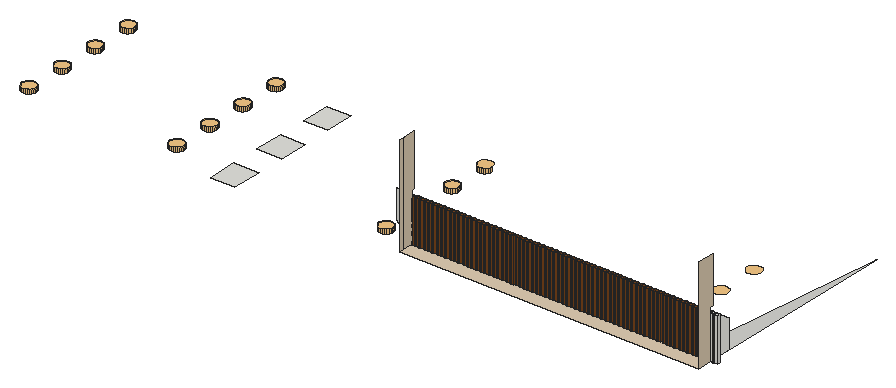
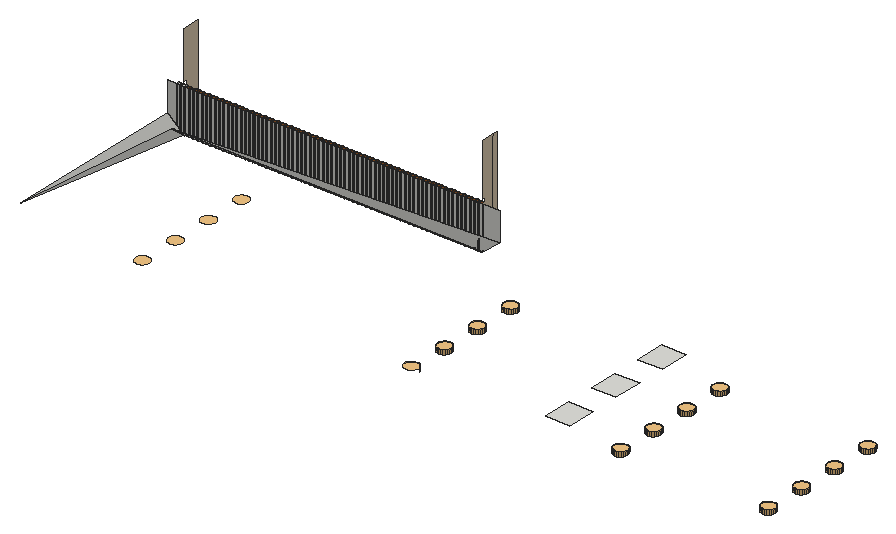
# SketchUp Ruby script. Lengths in inches.
U = 1.inch
M = Sketchup.active_model
def pt(a) = Geom::Point3d.new(a.map { |v| v * U })
def face(e, loops, mat)
  f = e.add_face(loops[0].map { |a| pt(a) })
  loops[1..].each { |l| e.add_face(l.map { |a| pt(a) }).erase! }
  f.material = f.back_material = mat if mat
  f
end
# faces: each face lists its corners as indices into pts; further lists are holes
def faces(e, pts, list, mat = nil) = list.each { |f| face(e, (f[0].is_a?(Array) ? f : [f]).map { |l| l.map { |i| pts[i] } }, mat) }
# xy, xz, yz: faces in a plane at the given z, y or x. An outline is a flat list of corners, or four numbers for a rectangle; further outlines are holes
def ring(l) = l.size == 4 ? [[l[0], l[1]], [l[2], l[1]], [l[2], l[3]], [l[0], l[3]]] : l.each_slice(2).to_a
def flat(e, list, mat, &to3) = list.each { |f| face(e, (f[0].is_a?(Array) ? f : [f]).map { |l| ring(l).map { |u, v| to3.(u, v) } }, mat) }
def xy(e, z, list, mat = nil) = flat(e, list, mat) { |x, y| [x, y, z] }
def xz(e, y, list, mat = nil) = flat(e, list, mat) { |x, z| [x, y, z] }
def yz(e, x, list, mat = nil) = flat(e, list, mat) { |y, z| [x, y, z] }
def lines(e, pts, list) = list.each { |a, b| e.add_line(pt(pts[a]), pt(pts[b])) }
# prism: a flat outline (further loops are holes) pulled along v
def prism(e, loops, v, mat = nil)
  f = face(e, loops, mat); d = Geom::Vector3d.new(v.map { |x| x * U })
  f.pushpull(f.normal.samedirection?(d) ? d.length : -d.length)
end
def box(e, o, s, mat = nil) = prism(e, [[o, [o[0] + s[0], o[1], o[2]], [o[0] + s[0], o[1] + s[1], o[2]], [o[0], o[1] + s[1], o[2]]]], [0, 0, s[2]], mat)
def at(x, y, z, deg = 0) = Geom::Transformation.translation(pt([x, y, z])) * Geom::Transformation.rotation(ORIGIN, Z_AXIS, deg.degrees)
def axes(o, x, y, z) = Geom::Transformation.new([*x, 0, *y, 0, *z, 0, *pt(o).to_a, 1])
def part(name) = M.definitions.add(name)
# library, detail: a bought-in or finely detailed component or shape, given as its bounding box
def library(name, o, s) = part(name).tap { |d| box(d.entities, o, s) }
def detail(e, o, s) = box(e.add_group.entities, o, s)
def put(e, d, t, mat = nil) = e.add_instance(d, t).tap { |i| i.material = mat if mat }
def group(e, t, mat = nil) = e.add_group.tap { |g| g.transformation = t; g.material = mat if mat }.entities
root = M.entities
M.materials.add("Generic\#1").color = [121, 68, 27]
M.materials.add("Generic\#2").color = [245, 199, 133]
M.materials.add("Generic\#6").color = [223, 205, 179]
c1 = part("Group\#11")
xy(c1.entities,26.3125,[[0,0,2,2]])
xz(c1.entities,0,[[0,0,2,26.3125]])
yz(c1.entities,0,[[0,0,2,26.3125]])
yz(c1.entities,2,[[0,0,2,26.3125]])
xy(root,122,[[190.6,57.81,205.29,75.37],[190.6,92.87,205.29,110.43],[190.6,127.93,205.29,145.49]])
xy(root,122.5625,[[68.07,68.72,66.98,68.86,65.97,69.28,65.11,69.95,64.44,70.8125,64.02,71.82,63.88,72.91,64.02,73.99,64.44,75,65.11,75.87,65.97,76.53,66.98,76.95,68.07,77.09,69.15,76.95,70.16,76.53,71.03,75.87,71.69,75,72.11,73.99,72.25,72.91,72.11,71.82,71.69,70.8125,71.03,69.95,70.16,69.28,69.15,68.86],[157.88,68.72,156.8,68.86,155.79,69.28,154.92,69.95,154.25,70.8125,153.83,71.82,153.69,72.91,153.83,73.99,154.25,75,154.92,75.87,155.79,76.53,156.8,76.95,157.88,77.09,158.96,76.95,159.97,76.53,160.84,75.87,161.51,75,161.92,73.99,162.07,72.91,161.92,71.82,161.51,70.8125,160.84,69.95,159.97,69.28,158.96,68.86],[284.88,68.72,283.8,68.86,282.79,69.28,281.92,69.95,281.25,70.8125,280.83,71.82,280.69,72.91,280.83,73.99,281.25,75,281.92,75.87,282.79,76.53,283.8,76.95,284.88,77.09,285.96,76.95,286.97,76.53,287.84,75.87,288.51,75,288.92,73.99,289.07,72.91,288.92,71.82,288.51,70.8125,287.84,69.95,286.97,69.28,285.96,68.86],[448.19,68.72,447.11,68.86,446.1,69.28,445.23,69.95,444.57,70.8125,444.15,71.82,444,72.91,444.15,73.99,444.57,75,445.23,75.87,446.1,76.53,447.11,76.95,448.19,77.09,449.28,76.95,450.29,76.53,451.15,75.87,451.82,75,452.24,73.99,452.38,72.91,452.24,71.82,451.82,70.8125,451.15,69.95,450.29,69.28,449.28,68.86],[68.07,93.78,66.98,93.92,65.97,94.34,65.11,95.01,64.44,95.875,64.02,96.89,63.88,97.97,64.02,99.05,64.44,100.0625,65.11,100.93,65.97,101.6,66.98,102.01,68.07,102.16,69.15,102.01,70.16,101.6,71.03,100.93,71.69,100.0625,72.11,99.05,72.25,97.97,72.11,96.89,71.69,95.875,71.03,95.01,70.16,94.34,69.15,93.92],
  [157.88,93.78,156.8,93.92,155.79,94.34,154.92,95.01,154.25,95.875,153.83,96.89,153.69,97.97,153.83,99.05,154.25,100.0625,154.92,100.93,155.79,101.6,156.8,102.01,157.88,102.16,158.96,102.01,159.97,101.6,160.84,100.93,161.51,100.0625,161.92,99.05,162.07,97.97,161.92,96.89,161.51,95.875,160.84,95.01,159.97,94.34,158.96,93.92],[284.88,93.78,283.8,93.92,282.79,94.34,281.92,95.01,281.25,95.875,280.83,96.89,280.69,97.97,280.83,99.05,281.25,100.0625,281.92,100.93,282.79,101.6,283.8,102.01,284.88,102.16,285.96,102.01,286.97,101.6,287.84,100.93,288.51,100.0625,288.92,99.05,289.07,97.97,288.92,96.89,288.51,95.875,287.84,95.01,286.97,94.34,285.96,93.92],[448.19,93.78,447.11,93.92,446.1,94.34,445.23,95.01,444.57,95.875,444.15,96.89,444,97.97,444.15,99.05,444.57,100.0625,445.23,100.93,446.1,101.6,447.11,102.01,448.19,102.16,449.28,102.01,450.29,101.6,451.15,100.93,451.82,100.0625,452.24,99.05,452.38,97.97,452.24,96.89,451.82,95.875,451.15,95.01,450.29,94.34,449.28,93.92],[68.07,118.84,66.98,118.99,65.97,119.41,65.11,120.07,64.44,120.9375,64.02,121.95,63.88,123.03,64.02,124.12,64.44,125.125,65.11,125.99,65.97,126.66,66.98,127.08,68.07,127.22,69.15,127.08,70.16,126.66,71.03,125.99,71.69,125.125,72.11,124.12,72.25,123.03,72.11,121.95,71.69,120.9375,71.03,120.07,70.16,119.41,69.15,118.99],[157.88,118.84,156.8,118.99,155.79,119.41,154.92,120.07,154.25,120.9375,153.83,121.95,153.69,123.03,153.83,124.12,154.25,125.125,154.92,125.99,155.79,126.66,156.8,127.08,157.88,127.22,158.96,127.08,159.97,126.66,160.84,125.99,161.51,125.125,161.92,124.12,162.07,123.03,161.92,121.95,161.51,120.9375,160.84,120.07,159.97,119.41,158.96,118.99],
  [284.88,118.84,283.8,118.99,282.79,119.41,281.92,120.07,281.25,120.9375,280.83,121.95,280.69,123.03,280.83,124.12,281.25,125.125,281.92,125.99,282.79,126.66,283.8,127.08,284.88,127.22,285.96,127.08,286.97,126.66,287.84,125.99,288.51,125.125,288.92,124.12,289.07,123.03,288.92,121.95,288.51,120.9375,287.84,120.07,286.97,119.41,285.96,118.99],[448.19,118.84,447.11,118.99,446.1,119.41,445.23,120.07,444.57,120.9375,444.15,121.95,444,123.03,444.15,124.12,444.57,125.125,445.23,125.99,446.1,126.66,447.11,127.08,448.19,127.22,449.28,127.08,450.29,126.66,451.15,125.99,451.82,125.125,452.24,124.12,452.38,123.03,452.24,121.95,451.82,120.9375,451.15,120.07,450.29,119.41,449.28,118.99],[68.07,143.91,66.98,144.05,65.97,144.47,65.11,145.13,64.44,146,64.02,147.01,63.88,148.09,64.02,149.18,64.44,150.1875,65.11,151.06,65.97,151.72,66.98,152.14,68.07,152.28,69.15,152.14,70.16,151.72,71.03,151.06,71.69,150.1875,72.11,149.18,72.25,148.09,72.11,147.01,71.69,146,71.03,145.13,70.16,144.47,69.15,144.05],[157.88,143.91,156.8,144.05,155.79,144.47,154.92,145.13,154.25,146,153.83,147.01,153.69,148.09,153.83,149.18,154.25,150.1875,154.92,151.06,155.79,151.72,156.8,152.14,157.88,152.28,158.96,152.14,159.97,151.72,160.84,151.06,161.51,150.1875,161.92,149.18,162.07,148.09,161.92,147.01,161.51,146,160.84,145.13,159.97,144.47,158.96,144.05],[284.88,143.91,283.8,144.05,282.79,144.47,281.92,145.13,281.25,146,280.83,147.01,280.69,148.09,280.83,149.18,281.25,150.1875,281.92,151.06,282.79,151.72,283.8,152.14,284.88,152.28,285.96,152.14,286.97,151.72,287.84,151.06,288.51,150.1875,288.92,149.18,289.07,148.09,288.92,147.01,288.51,146,287.84,145.13,286.97,144.47,285.96,144.05],
  [448.19,143.91,447.11,144.05,446.1,144.47,445.23,145.13,444.57,146,444.15,147.01,444,148.09,444.15,149.18,444.57,150.1875,445.23,151.06,446.1,151.72,447.11,152.14,448.19,152.28,449.28,152.14,450.29,151.72,451.15,151.06,451.82,150.1875,452.24,149.18,452.38,148.09,452.24,147.01,451.82,146,451.15,145.13,450.29,144.47,449.28,144.05]],"Generic\#2")
xy(root,132.125,[[316.59,43.625,497.875,54.5625]],"Generic\#6")
xz(root,54.5625,[[316.59,132.125,316.59,158.4375,306.09,158.4375,306.09,140.875],[316.59,132.125,318.59,158.4375],[318.59,132.125,497.875,158.4375],[497.875,132.125,507.875,140.875,507.875,158.4375,497.875,158.4375]])
yz(root,316.59,[[43.625,132.125,46.4375,192.9375],[46.4375,132.125,54.5625,132.125,54.5625,158.4375,52.5625,158.4375,52.5625,161.25,54.5625,161.25,54.5625,192.9375,46.4375,192.9375]],"Generic\#6")
yz(root,497.875,[[43.625,132.125,43.625,189.99,54.5625,189.99,54.5625,161.25,52.5625,161.25,52.5625,158.4375,54.5625,158.4375,54.5625,132.125]],"Generic\#6")
p = [[68.07,68.72,120],[66.98,68.86,120],[66.98,68.86,122.5625],[68.07,68.72,122.5625],[69.15,68.86,120],[69.15,68.86,122.5625],
  [157.88,68.72,120],[156.8,68.86,120],[156.8,68.86,122.5625],[157.88,68.72,122.5625],[158.96,68.86,120],[158.96,68.86,122.5625],
  [284.88,68.72,120],[283.8,68.86,120],[283.8,68.86,122.5625],[284.88,68.72,122.5625],[285.96,68.86,120],[285.96,68.86,122.5625],
  [65.97,69.28,120],[65.97,69.28,122.5625],[70.16,69.28,120],[70.16,69.28,122.5625],[155.79,69.28,120],[155.79,69.28,122.5625],
  [159.97,69.28,120],[159.97,69.28,122.5625],[282.79,69.28,120],[282.79,69.28,122.5625],[286.97,69.28,120],[286.97,69.28,122.5625],
  [65.11,69.95,120],[65.11,69.95,122.5625],[71.03,69.95,120],[71.03,69.95,122.5625],[154.92,69.95,120],[154.92,69.95,122.5625],
  [160.84,69.95,120],[160.84,69.95,122.5625],[281.92,69.95,120],[281.92,69.95,122.5625],[287.84,69.95,120],[287.84,69.95,122.5625],
  [64.44,70.8125,120],[64.44,70.8125,122.5625],[71.69,70.8125,120],[71.69,70.8125,122.5625],[154.25,70.8125,120],[154.25,70.8125,122.5625],
  [161.51,70.8125,120],[161.51,70.8125,122.5625],[281.25,70.8125,120],[281.25,70.8125,122.5625],[288.51,70.8125,120],[288.51,70.8125,122.5625],
  [64.02,71.82,120],[64.02,71.82,122.5625],[72.11,71.82,120],[72.11,71.82,122.5625],[153.83,71.82,120],[153.83,71.82,122.5625],
  [161.92,71.82,120],[161.92,71.82,122.5625],[280.83,71.82,120],[280.83,71.82,122.5625],[288.92,71.82,120],[288.92,71.82,122.5625],
  [63.88,72.91,120],[63.88,72.91,122.5625],[72.25,72.91,120],[72.25,72.91,122.5625],[153.69,72.91,120],[153.69,72.91,122.5625],
  [162.07,72.91,120],[162.07,72.91,122.5625],[280.69,72.91,120],[280.69,72.91,122.5625],[289.07,72.91,120],[289.07,72.91,122.5625],
  [64.02,73.99,120],[64.02,73.99,122.5625],[72.11,73.99,120],[72.11,73.99,122.5625],[153.83,73.99,120],[153.83,73.99,122.5625],
  [161.92,73.99,120],[161.92,73.99,122.5625],[280.83,73.99,120],[280.83,73.99,122.5625],[288.92,73.99,120],[288.92,73.99,122.5625],
  [64.44,75,120],[64.44,75,122.5625],[71.69,75,120],[71.69,75,122.5625],[154.25,75,120],[154.25,75,122.5625],
  [161.51,75,120],[161.51,75,122.5625],[281.25,75,120],[281.25,75,122.5625],[288.51,75,120],[288.51,75,122.5625],
  [65.11,75.87,120],[65.11,75.87,122.5625],[71.03,75.87,120],[71.03,75.87,122.5625],[154.92,75.87,120],[154.92,75.87,122.5625],
  [160.84,75.87,120],[160.84,75.87,122.5625],[281.92,75.87,120],[281.92,75.87,122.5625],[287.84,75.87,120],[287.84,75.87,122.5625],
  [65.97,76.53,120],[65.97,76.53,122.5625],[70.16,76.53,120],[70.16,76.53,122.5625],[155.79,76.53,120],[155.79,76.53,122.5625],
  [159.97,76.53,120],[159.97,76.53,122.5625],[282.79,76.53,120],[282.79,76.53,122.5625],[286.97,76.53,120],[286.97,76.53,122.5625],
  [66.98,76.95,120],[66.98,76.95,122.5625],[69.15,76.95,120],[69.15,76.95,122.5625],[156.8,76.95,120],[156.8,76.95,122.5625],
  [158.96,76.95,120],[158.96,76.95,122.5625],[283.8,76.95,120],[283.8,76.95,122.5625],[285.96,76.95,120],[285.96,76.95,122.5625],
  [68.07,77.09,120],[68.07,77.09,122.5625],[157.88,77.09,120],[157.88,77.09,122.5625],[284.88,77.09,120],[284.88,77.09,122.5625],
  [68.07,93.78,120],[66.98,93.92,120],[66.98,93.92,122.5625],[68.07,93.78,122.5625],[69.15,93.92,120],[69.15,93.92,122.5625],
  [157.88,93.78,120],[156.8,93.92,120],[156.8,93.92,122.5625],[157.88,93.78,122.5625],[158.96,93.92,120],[158.96,93.92,122.5625],
  [284.88,93.78,120],[283.8,93.92,120],[283.8,93.92,122.5625],[284.88,93.78,122.5625],[285.96,93.92,120],[285.96,93.92,122.5625],
  [65.97,94.34,120],[65.97,94.34,122.5625],[70.16,94.34,120],[70.16,94.34,122.5625],[155.79,94.34,120],[155.79,94.34,122.5625],
  [159.97,94.34,120],[159.97,94.34,122.5625],[282.79,94.34,120],[282.79,94.34,122.5625],[286.97,94.34,120],[286.97,94.34,122.5625],
  [65.11,95.01,120],[65.11,95.01,122.5625],[71.03,95.01,120],[71.03,95.01,122.5625],[154.92,95.01,120],[154.92,95.01,122.5625],
  [160.84,95.01,120],[160.84,95.01,122.5625],[281.92,95.01,120],[281.92,95.01,122.5625],[287.84,95.01,120],[287.84,95.01,122.5625],
  [64.44,95.875,120],[64.44,95.875,122.5625],[71.69,95.875,120],[71.69,95.875,122.5625],[154.25,95.875,120],[154.25,95.875,122.5625],
  [161.51,95.875,120],[161.51,95.875,122.5625],[281.25,95.875,120],[281.25,95.875,122.5625],[288.51,95.875,120],[288.51,95.875,122.5625],
  [64.02,96.89,120],[64.02,96.89,122.5625],[72.11,96.89,120],[72.11,96.89,122.5625],[153.83,96.89,120],[153.83,96.89,122.5625],
  [161.92,96.89,120],[161.92,96.89,122.5625],[280.83,96.89,120],[280.83,96.89,122.5625],[288.92,96.89,120],[288.92,96.89,122.5625],
  [63.88,97.97,120],[63.88,97.97,122.5625],[72.25,97.97,120],[72.25,97.97,122.5625],[153.69,97.97,120],[153.69,97.97,122.5625],
  [162.07,97.97,120],[162.07,97.97,122.5625],[280.69,97.97,120],[280.69,97.97,122.5625],[289.07,97.97,120],[289.07,97.97,122.5625],
  [64.02,99.05,120],[64.02,99.05,122.5625],[72.11,99.05,120],[72.11,99.05,122.5625],[153.83,99.05,120],[153.83,99.05,122.5625],
  [161.92,99.05,120],[161.92,99.05,122.5625],[280.83,99.05,120],[280.83,99.05,122.5625],[288.92,99.05,120],[288.92,99.05,122.5625],
  [64.44,100.0625,120],[64.44,100.0625,122.5625],[71.69,100.0625,120],[71.69,100.0625,122.5625],[154.25,100.0625,120],[154.25,100.0625,122.5625],
  [161.51,100.0625,120],[161.51,100.0625,122.5625],[281.25,100.0625,120],[281.25,100.0625,122.5625],[288.51,100.0625,120],[288.51,100.0625,122.5625],
  [65.11,100.93,120],[65.11,100.93,122.5625],[71.03,100.93,120],[71.03,100.93,122.5625],[154.92,100.93,120],[154.92,100.93,122.5625],
  [160.84,100.93,120],[160.84,100.93,122.5625],[281.92,100.93,120],[281.92,100.93,122.5625],[287.84,100.93,120],[287.84,100.93,122.5625],
  [65.97,101.6,120],[65.97,101.6,122.5625],[70.16,101.6,120],[70.16,101.6,122.5625],[155.79,101.6,120],[155.79,101.6,122.5625],
  [159.97,101.6,120],[159.97,101.6,122.5625],[282.79,101.6,120],[282.79,101.6,122.5625],[286.97,101.6,120],[286.97,101.6,122.5625],
  [66.98,102.01,120],[66.98,102.01,122.5625],[69.15,102.01,120],[69.15,102.01,122.5625],[156.8,102.01,120],[156.8,102.01,122.5625],
  [158.96,102.01,120],[158.96,102.01,122.5625],[283.8,102.01,120],[283.8,102.01,122.5625],[285.96,102.01,120],[285.96,102.01,122.5625],
  [68.07,102.16,120],[68.07,102.16,122.5625],[157.88,102.16,120],[157.88,102.16,122.5625],[284.88,102.16,120],[284.88,102.16,122.5625],
  [68.07,118.84,120],[66.98,118.99,120],[66.98,118.99,122.5625],[68.07,118.84,122.5625],[69.15,118.99,120],[69.15,118.99,122.5625],
  [157.88,118.84,120],[156.8,118.99,120],[156.8,118.99,122.5625],[157.88,118.84,122.5625],[158.96,118.99,120],[158.96,118.99,122.5625],
  [284.88,118.84,120],[283.8,118.99,120],[283.8,118.99,122.5625],[284.88,118.84,122.5625],[285.96,118.99,120],[285.96,118.99,122.5625],
  [65.97,119.41,120],[65.97,119.41,122.5625],[70.16,119.41,120],[70.16,119.41,122.5625],[155.79,119.41,120],[155.79,119.41,122.5625],
  [159.97,119.41,120],[159.97,119.41,122.5625],[282.79,119.41,120],[282.79,119.41,122.5625],[286.97,119.41,120],[286.97,119.41,122.5625],
  [65.11,120.07,120],[65.11,120.07,122.5625],[71.03,120.07,120],[71.03,120.07,122.5625],[154.92,120.07,120],[154.92,120.07,122.5625],
  [160.84,120.07,120],[160.84,120.07,122.5625],[281.92,120.07,120],[281.92,120.07,122.5625],[287.84,120.07,120],[287.84,120.07,122.5625],
  [64.44,120.9375,120],[64.44,120.9375,122.5625],[71.69,120.9375,120],[71.69,120.9375,122.5625],[154.25,120.9375,120],[154.25,120.9375,122.5625],
  [161.51,120.9375,120],[161.51,120.9375,122.5625],[281.25,120.9375,120],[281.25,120.9375,122.5625],[288.51,120.9375,120],[288.51,120.9375,122.5625],
  [64.02,121.95,120],[64.02,121.95,122.5625],[72.11,121.95,120],[72.11,121.95,122.5625],[153.83,121.95,120],[153.83,121.95,122.5625],
  [161.92,121.95,120],[161.92,121.95,122.5625],[280.83,121.95,120],[280.83,121.95,122.5625],[288.92,121.95,120],[288.92,121.95,122.5625],
  [63.88,123.03,120],[63.88,123.03,122.5625],[72.25,123.03,120],[72.25,123.03,122.5625],[153.69,123.03,120],[153.69,123.03,122.5625],
  [162.07,123.03,120],[162.07,123.03,122.5625],[280.69,123.03,120],[280.69,123.03,122.5625],[289.07,123.03,120],[289.07,123.03,122.5625],
  [64.02,124.12,120],[64.02,124.12,122.5625],[72.11,124.12,120],[72.11,124.12,122.5625],[153.83,124.12,120],[153.83,124.12,122.5625],
  [161.92,124.12,120],[161.92,124.12,122.5625],[280.83,124.12,120],[280.83,124.12,122.5625],[288.92,124.12,120],[288.92,124.12,122.5625],
  [64.44,125.125,120],[64.44,125.125,122.5625],[71.69,125.125,120],[71.69,125.125,122.5625],[154.25,125.125,120],[154.25,125.125,122.5625],
  [161.51,125.125,120],[161.51,125.125,122.5625],[281.25,125.125,120],[281.25,125.125,122.5625],[288.51,125.125,120],[288.51,125.125,122.5625],
  [65.11,125.99,120],[65.11,125.99,122.5625],[71.03,125.99,120],[71.03,125.99,122.5625],[154.92,125.99,120],[154.92,125.99,122.5625],
  [160.84,125.99,120],[160.84,125.99,122.5625],[281.92,125.99,120],[281.92,125.99,122.5625],[287.84,125.99,120],[287.84,125.99,122.5625],
  [65.97,126.66,120],[65.97,126.66,122.5625],[70.16,126.66,120],[70.16,126.66,122.5625],[155.79,126.66,120],[155.79,126.66,122.5625],
  [159.97,126.66,120],[159.97,126.66,122.5625],[282.79,126.66,120],[282.79,126.66,122.5625],[286.97,126.66,120],[286.97,126.66,122.5625],
  [66.98,127.08,120],[66.98,127.08,122.5625],[69.15,127.08,120],[69.15,127.08,122.5625],[156.8,127.08,120],[156.8,127.08,122.5625],
  [158.96,127.08,120],[158.96,127.08,122.5625],[283.8,127.08,120],[283.8,127.08,122.5625],[285.96,127.08,120],[285.96,127.08,122.5625],
  [68.07,127.22,120],[68.07,127.22,122.5625],[157.88,127.22,120],[157.88,127.22,122.5625],[284.88,127.22,120],[284.88,127.22,122.5625],
  [68.07,143.91,120],[66.98,144.05,120],[66.98,144.05,122.5625],[68.07,143.91,122.5625],[69.15,144.05,120],[69.15,144.05,122.5625],
  [157.88,143.91,120],[156.8,144.05,120],[156.8,144.05,122.5625],[157.88,143.91,122.5625],[158.96,144.05,120],[158.96,144.05,122.5625],
  [284.88,143.91,120],[283.8,144.05,120],[283.8,144.05,122.5625],[284.88,143.91,122.5625],[285.96,144.05,120],[285.96,144.05,122.5625],
  [65.97,144.47,120],[65.97,144.47,122.5625],[70.16,144.47,120],[70.16,144.47,122.5625],[155.79,144.47,120],[155.79,144.47,122.5625],
  [159.97,144.47,120],[159.97,144.47,122.5625],[282.79,144.47,120],[282.79,144.47,122.5625],[286.97,144.47,120],[286.97,144.47,122.5625],
  [65.11,145.13,120],[65.11,145.13,122.5625],[71.03,145.13,120],[71.03,145.13,122.5625],[154.92,145.13,120],[154.92,145.13,122.5625],
  [160.84,145.13,120],[160.84,145.13,122.5625],[281.92,145.13,120],[281.92,145.13,122.5625],[287.84,145.13,120],[287.84,145.13,122.5625],
  [64.44,146,120],[64.44,146,122.5625],[71.69,146,120],[71.69,146,122.5625],[154.25,146,120],[154.25,146,122.5625],
  [161.51,146,120],[161.51,146,122.5625],[281.25,146,120],[281.25,146,122.5625],[288.51,146,120],[288.51,146,122.5625],
  [64.02,147.01,120],[64.02,147.01,122.5625],[72.11,147.01,120],[72.11,147.01,122.5625],[153.83,147.01,120],[153.83,147.01,122.5625],
  [161.92,147.01,120],[161.92,147.01,122.5625],[280.83,147.01,120],[280.83,147.01,122.5625],[288.92,147.01,120],[288.92,147.01,122.5625],
  [63.88,148.09,120],[63.88,148.09,122.5625],[72.25,148.09,120],[72.25,148.09,122.5625],[153.69,148.09,120],[153.69,148.09,122.5625],
  [162.07,148.09,120],[162.07,148.09,122.5625],[289.07,148.09,120],[289.07,148.09,122.5625],[64.02,149.18,120],[64.02,149.18,122.5625],
  [72.11,149.18,120],[72.11,149.18,122.5625],[153.83,149.18,120],[153.83,149.18,122.5625],[161.92,149.18,120],[161.92,149.18,122.5625],
  [64.44,150.1875,120],[64.44,150.1875,122.5625],[71.69,150.1875,120],[71.69,150.1875,122.5625],[154.25,150.1875,120],[154.25,150.1875,122.5625],
  [161.51,150.1875,120],[161.51,150.1875,122.5625],[65.11,151.06,120],[65.11,151.06,122.5625],[71.03,151.06,120],[71.03,151.06,122.5625],
  [154.92,151.06,120],[154.92,151.06,122.5625],[160.84,151.06,120],[160.84,151.06,122.5625],[65.97,151.72,120],[65.97,151.72,122.5625],
  [70.16,151.72,120],[70.16,151.72,122.5625],[155.79,151.72,120],[155.79,151.72,122.5625],[159.97,151.72,120],[159.97,151.72,122.5625],
  [66.98,152.14,120],[66.98,152.14,122.5625],[69.15,152.14,120],[69.15,152.14,122.5625],[156.8,152.14,120],[156.8,152.14,122.5625],
  [158.96,152.14,120],[158.96,152.14,122.5625],[68.07,152.28,120],[68.07,152.28,122.5625],[157.88,152.28,120],[157.88,152.28,122.5625],
  [316.59,54.5625,132.125],[306.09,54.5625,140.875],[496.1875,65.5625,140.875],[318.59,54.5625,132.125],[497.875,54.5625,132.125],[507.875,166.1875,140.875],
  [507.875,54.5625,140.875],[318.59,52.5625,132.125]]
faces(root,p,[[0,1,2,3],[4,0,3,5],[6,7,8,9],[10,6,9,11],[12,13,14,15],[16,12,15,17],[1,18,19,2],[20,4,5,21],
  [7,22,23,8],[24,10,11,25],[13,26,27,14],[28,16,17,29],[18,30,31,19],[32,20,21,33],[22,34,35,23],[36,24,25,37],
  [26,38,39,27],[40,28,29,41],[30,42,43,31],[44,32,33,45],[34,46,47,35],[48,36,37,49],[38,50,51,39],[52,40,41,53],
  [42,54,55,43],[56,44,45,57],[46,58,59,47],[60,48,49,61],[50,62,63,51],[64,52,53,65],[54,66,67,55],[68,56,57,69],
  [58,70,71,59],[72,60,61,73],[62,74,75,63],[76,64,65,77],[66,78,79,67],[80,68,69,81],[70,82,83,71],[84,72,73,85],
  [74,86,87,75],[88,76,77,89],[78,90,91,79],[92,80,81,93],[82,94,95,83],[96,84,85,97],[86,98,99,87],[100,88,89,101],
  [90,102,103,91],[104,92,93,105],[94,106,107,95],[108,96,97,109],[98,110,111,99],[112,100,101,113],[102,114,115,103],[116,104,105,117],
  [106,118,119,107],[120,108,109,121],[110,122,123,111],[124,112,113,125],[114,126,127,115],[128,116,117,129],[118,130,131,119],[132,120,121,133],
  [122,134,135,123],[136,124,125,137],[126,138,139,127],[138,128,129,139],[130,140,141,131],[140,132,133,141],[134,142,143,135],[142,136,137,143],
  [144,145,146,147],[148,144,147,149],[150,151,152,153],[154,150,153,155],[156,157,158,159],[160,156,159,161],[145,162,163,146],[164,148,149,165],
  [151,166,167,152],[168,154,155,169],[157,170,171,158],[172,160,161,173],[162,174,175,163],[176,164,165,177],[166,178,179,167],[180,168,169,181],
  [170,182,183,171],[184,172,173,185],[174,186,187,175],[188,176,177,189],[178,190,191,179],[192,180,181,193],[182,194,195,183],[196,184,185,197],
  [186,198,199,187],[200,188,189,201],[190,202,203,191],[204,192,193,205],[194,206,207,195],[208,196,197,209],[198,210,211,199],[212,200,201,213],
  [202,214,215,203],[216,204,205,217],[206,218,219,207],[220,208,209,221],[210,222,223,211],[224,212,213,225],[214,226,227,215],[228,216,217,229],
  [218,230,231,219],[232,220,221,233],[222,234,235,223],[236,224,225,237],[226,238,239,227],[240,228,229,241],[230,242,243,231],[244,232,233,245],
  [234,246,247,235],[248,236,237,249],[238,250,251,239],[252,240,241,253],[242,254,255,243],[256,244,245,257],[246,258,259,247],[260,248,249,261],
  [250,262,263,251],[264,252,253,265],[254,266,267,255],[268,256,257,269],[258,270,271,259],[272,260,261,273],[262,274,275,263],[276,264,265,277],
  [266,278,279,267],[280,268,269,281],[270,282,283,271],[282,272,273,283],[274,284,285,275],[284,276,277,285],[278,286,287,279],[286,280,281,287],
  [288,289,290,291],[292,288,291,293],[294,295,296,297],[298,294,297,299],[300,301,302,303],[304,300,303,305],[289,306,307,290],[308,292,293,309],
  [295,310,311,296],[312,298,299,313],[301,314,315,302],[316,304,305,317],[306,318,319,307],[320,308,309,321],[310,322,323,311],[324,312,313,325],
  [314,326,327,315],[328,316,317,329],[318,330,331,319],[332,320,321,333],[322,334,335,323],[336,324,325,337],[326,338,339,327],[340,328,329,341],
  [330,342,343,331],[344,332,333,345],[334,346,347,335],[348,336,337,349],[338,350,351,339],[352,340,341,353],[342,354,355,343],[356,344,345,357],
  [346,358,359,347],[360,348,349,361],[350,362,363,351],[364,352,353,365],[354,366,367,355],[368,356,357,369],[358,370,371,359],[372,360,361,373],
  [362,374,375,363],[376,364,365,377],[366,378,379,367],[380,368,369,381],[370,382,383,371],[384,372,373,385],[374,386,387,375],[388,376,377,389],
  [378,390,391,379],[392,380,381,393],[382,394,395,383],[396,384,385,397],[386,398,399,387],[400,388,389,401],[390,402,403,391],[404,392,393,405],
  [394,406,407,395],[408,396,397,409],[398,410,411,399],[412,400,401,413],[402,414,415,403],[416,404,405,417],[406,418,419,407],[420,408,409,421],
  [410,422,423,411],[424,412,413,425],[414,426,427,415],[426,416,417,427],[418,428,429,419],[428,420,421,429],[422,430,431,423],[430,424,425,431],
  [432,433,434,435],[436,432,435,437],[438,439,440,441],[442,438,441,443],[444,445,446,447],[448,444,447,449],[433,450,451,434],[452,436,437,453],
  [439,454,455,440],[456,442,443,457],[445,458,459,446],[460,448,449,461],[450,462,463,451],[464,452,453,465],[454,466,467,455],[468,456,457,469],
  [458,470,471,459],[472,460,461,473],[462,474,475,463],[476,464,465,477],[466,478,479,467],[480,468,469,481],[470,482,483,471],[484,472,473,485],
  [474,486,487,475],[488,476,477,489],[478,490,491,479],[492,480,481,493],[482,494,495,483],[496,484,485,497],[486,498,499,487],[500,488,489,501],
  [490,502,503,491],[504,492,493,505],[506,496,497,507],[498,508,509,499],[510,500,501,511],[502,512,513,503],[514,504,505,515],[508,516,517,509],
  [518,510,511,519],[512,520,521,513],[522,514,515,523],[516,524,525,517],[526,518,519,527],[520,528,529,521],[530,522,523,531],[524,532,533,525],
  [534,526,527,535],[528,536,537,529],[538,530,531,539],[532,540,541,533],[542,534,535,543],[536,544,545,537],[546,538,539,547],[540,548,549,541],
  [548,542,543,549],[544,550,551,545],[550,546,547,551]],"Generic\#2")
faces(root,p,[[552,553,554],[555,552,554,556],[556,554,557],[558,556,557]])
lines(root,p,[[555,559]])
put(root,c1,at(316.59,52.5625,132.125),"Generic\#1")
put(root,c1,at(319.22,52.5625,132.125),"Generic\#1")
put(root,c1,at(321.84,52.5625,132.125),"Generic\#1")
put(root,c1,at(324.47,52.5625,132.125),"Generic\#1")
put(root,c1,at(327.09,52.5625,132.125),"Generic\#1")
put(root,c1,at(329.72,52.5625,132.125),"Generic\#1")
put(root,c1,at(332.34,52.5625,132.125),"Generic\#1")
put(root,c1,at(334.97,52.5625,132.125),"Generic\#1")
put(root,c1,at(337.59,52.5625,132.125),"Generic\#1")
put(root,c1,at(340.22,52.5625,132.125),"Generic\#1")
put(root,c1,at(342.84,52.5625,132.125),"Generic\#1")
put(root,c1,at(345.47,52.5625,132.125),"Generic\#1")
put(root,c1,at(348.09,52.5625,132.125),"Generic\#1")
put(root,c1,at(350.72,52.5625,132.125),"Generic\#1")
put(root,c1,at(353.34,52.5625,132.125),"Generic\#1")
put(root,c1,at(355.97,52.5625,132.125),"Generic\#1")
put(root,c1,at(358.59,52.5625,132.125),"Generic\#1")
put(root,c1,at(361.22,52.5625,132.125),"Generic\#1")
put(root,c1,at(363.84,52.5625,132.125),"Generic\#1")
put(root,c1,at(366.47,52.5625,132.125),"Generic\#1")
put(root,c1,at(369.09,52.5625,132.125),"Generic\#1")
put(root,c1,at(371.72,52.5625,132.125),"Generic\#1")
put(root,c1,at(374.34,52.5625,132.125),"Generic\#1")
put(root,c1,at(376.97,52.5625,132.125),"Generic\#1")
put(root,c1,at(379.59,52.5625,132.125),"Generic\#1")
put(root,c1,at(382.22,52.5625,132.125),"Generic\#1")
put(root,c1,at(384.84,52.5625,132.125),"Generic\#1")
put(root,c1,at(387.47,52.5625,132.125),"Generic\#1")
put(root,c1,at(390.09,52.5625,132.125),"Generic\#1")
put(root,c1,at(392.72,52.5625,132.125),"Generic\#1")
put(root,c1,at(395.34,52.5625,132.125),"Generic\#1")
put(root,c1,at(397.97,52.5625,132.125),"Generic\#1")
put(root,c1,at(400.59,52.5625,132.125),"Generic\#1")
put(root,c1,at(403.22,52.5625,132.125),"Generic\#1")
put(root,c1,at(405.84,52.5625,132.125),"Generic\#1")
put(root,c1,at(408.47,52.5625,132.125),"Generic\#1")
put(root,c1,at(411.09,52.5625,132.125),"Generic\#1")
put(root,c1,at(413.72,52.5625,132.125),"Generic\#1")
put(root,c1,at(416.34,52.5625,132.125),"Generic\#1")
put(root,c1,at(418.97,52.5625,132.125),"Generic\#1")
put(root,c1,at(421.59,52.5625,132.125),"Generic\#1")
put(root,c1,at(424.22,52.5625,132.125),"Generic\#1")
put(root,c1,at(426.84,52.5625,132.125),"Generic\#1")
put(root,c1,at(429.47,52.5625,132.125),"Generic\#1")
put(root,c1,at(432.09,52.5625,132.125),"Generic\#1")
put(root,c1,at(434.72,52.5625,132.125),"Generic\#1")
put(root,c1,at(437.34,52.5625,132.125),"Generic\#1")
put(root,c1,at(439.97,52.5625,132.125),"Generic\#1")
put(root,c1,at(442.59,52.5625,132.125),"Generic\#1")
put(root,c1,at(445.22,52.5625,132.125),"Generic\#1")
put(root,c1,at(447.84,52.5625,132.125),"Generic\#1")
put(root,c1,at(450.47,52.5625,132.125),"Generic\#1")
put(root,c1,at(453.09,52.5625,132.125),"Generic\#1")
put(root,c1,at(455.72,52.5625,132.125),"Generic\#1")
put(root,c1,at(458.34,52.5625,132.125),"Generic\#1")
put(root,c1,at(460.97,52.5625,132.125),"Generic\#1")
put(root,c1,at(463.59,52.5625,132.125),"Generic\#1")
put(root,c1,at(466.22,52.5625,132.125),"Generic\#1")
put(root,c1,at(468.84,52.5625,132.125),"Generic\#1")
put(root,c1,at(471.47,52.5625,132.125),"Generic\#1")
put(root,c1,at(474.09,52.5625,132.125),"Generic\#1")
put(root,c1,at(476.72,52.5625,132.125),"Generic\#1")
put(root,c1,at(479.34,52.5625,132.125),"Generic\#1")
put(root,c1,at(481.97,52.5625,132.125),"Generic\#1")
put(root,c1,at(484.59,52.5625,132.125),"Generic\#1")
put(root,c1,at(487.22,52.5625,132.125),"Generic\#1")
put(root,c1,at(489.84,52.5625,132.125),"Generic\#1")
put(root,c1,at(492.47,52.5625,132.125),"Generic\#1")
put(root,c1,at(495.09,52.5625,132.125),"Generic\#1")
put(root,c1,at(497.72,52.5625,132.125))
put(root,c1,at(500.34,52.5625,132.125))
